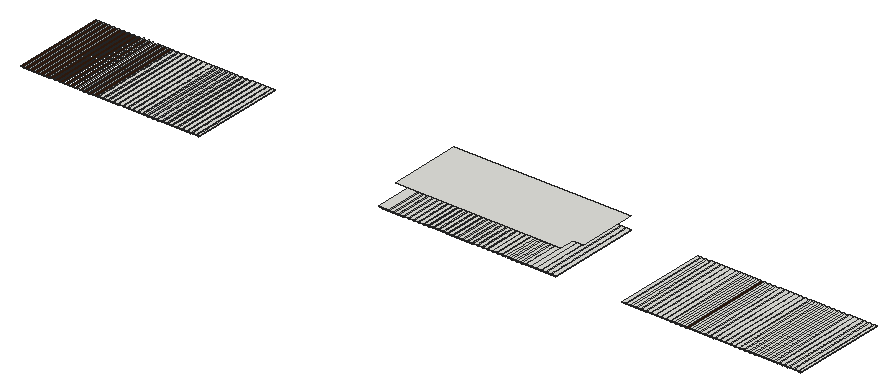
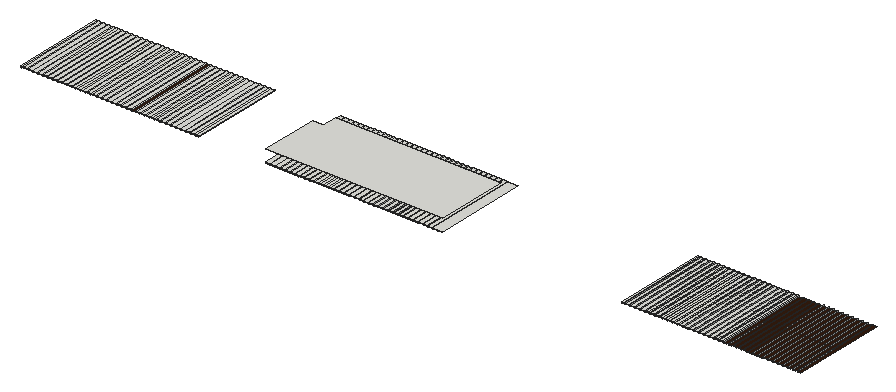
# SketchUp Ruby script. Lengths in inches.
U = 1.inch
M = Sketchup.active_model
def pt(a) = Geom::Point3d.new(a.map { |v| v * U })
def face(e, loops, mat)
  f = e.add_face(loops[0].map { |a| pt(a) })
  loops[1..].each { |l| e.add_face(l.map { |a| pt(a) }).erase! }
  f.material = f.back_material = mat if mat
  f
end
# faces: each face lists its corners as indices into pts; further lists are holes
def faces(e, pts, list, mat = nil) = list.each { |f| face(e, (f[0].is_a?(Array) ? f : [f]).map { |l| l.map { |i| pts[i] } }, mat) }
# xy, xz, yz: faces in a plane at the given z, y or x. An outline is a flat list of corners, or four numbers for a rectangle; further outlines are holes
def ring(l) = l.size == 4 ? [[l[0], l[1]], [l[2], l[1]], [l[2], l[3]], [l[0], l[3]]] : l.each_slice(2).to_a
def flat(e, list, mat, &to3) = list.each { |f| face(e, (f[0].is_a?(Array) ? f : [f]).map { |l| ring(l).map { |u, v| to3.(u, v) } }, mat) }
def xy(e, z, list, mat = nil) = flat(e, list, mat) { |x, y| [x, y, z] }
def xz(e, y, list, mat = nil) = flat(e, list, mat) { |x, z| [x, y, z] }
def yz(e, x, list, mat = nil) = flat(e, list, mat) { |y, z| [x, y, z] }
def lines(e, pts, list) = list.each { |a, b| e.add_line(pt(pts[a]), pt(pts[b])) }
# prism: a flat outline (further loops are holes) pulled along v
def prism(e, loops, v, mat = nil)
  f = face(e, loops, mat); d = Geom::Vector3d.new(v.map { |x| x * U })
  f.pushpull(f.normal.samedirection?(d) ? d.length : -d.length)
end
def box(e, o, s, mat = nil) = prism(e, [[o, [o[0] + s[0], o[1], o[2]], [o[0] + s[0], o[1] + s[1], o[2]], [o[0], o[1] + s[1], o[2]]]], [0, 0, s[2]], mat)
def at(x, y, z, deg = 0) = Geom::Transformation.translation(pt([x, y, z])) * Geom::Transformation.rotation(ORIGIN, Z_AXIS, deg.degrees)
def axes(o, x, y, z) = Geom::Transformation.new([*x, 0, *y, 0, *z, 0, *pt(o).to_a, 1])
def part(name) = M.definitions.add(name)
# library, detail: a bought-in or finely detailed component or shape, given as its bounding box
def library(name, o, s) = part(name).tap { |d| box(d.entities, o, s) }
def detail(e, o, s) = box(e.add_group.entities, o, s)
def put(e, d, t, mat = nil) = e.add_instance(d, t).tap { |i| i.material = mat if mat }
def group(e, t, mat = nil) = e.add_group.tap { |g| g.transformation = t; g.material = mat if mat }.entities
root = M.entities
M.materials.add("[Wood Veneer 01]").color = [51, 28, 15]
xy(root,253.5625,[[1723.81,246.64,1728.56,361.27],[1729.81,246.64,1734.56,361.27],[1735.81,246.64,1740.56,361.27],[1741.81,246.64,1746.56,361.27],[1747.81,246.64,1752.56,361.27],
  [1753.81,246.64,1758.56,361.27],[1759.81,246.64,1764.56,361.27],[1765.81,246.64,1770.56,361.27],[1771.81,246.64,1776.56,361.27],[1777.81,246.64,1782.56,361.27]],"[Wood Veneer 01]")
xy(root,253.875,[[1711.81,246.64,1716.56,361.27],[1717.81,246.64,1722.56,361.27]],"[Wood Veneer 01]")
xy(root,253.9375,[[1130.14,246.64,1134.52,361.27],[1136.14,246.64,1140.52,361.27],[1142.14,246.64,1146.52,361.27],[1148.14,246.64,1152.52,361.27],[1154.14,246.64,1158.52,361.27],
  [1160.14,246.64,1164.52,361.27],[1166.14,246.64,1170.52,361.27],[1172.14,246.64,1176.52,361.27],[1178.14,246.64,1182.52,361.27],[1184.14,246.64,1188.52,361.27],
  [1190.14,246.64,1194.52,361.27],[1196.14,246.64,1200.52,361.27],[1202.14,246.64,1206.52,361.27],[1208.14,246.64,1212.52,361.27],[1214.14,246.64,1218.52,361.27],
  [1220.14,246.64,1224.52,361.27],[1226.14,246.64,1230.52,361.27],[1232.14,246.64,1236.52,361.27],[1238.14,246.64,1242.52,361.27],[1244.14,246.64,1248.52,361.27],
  [1250.14,246.64,1254.52,361.27],[1256.14,246.64,1260.52,361.27],[1262.14,246.64,1266.52,361.27],[1268.14,246.64,1272.52,361.27],[1274.14,246.64,1278.52,361.27],
  [1280.14,246.64,1284.52,361.27],[1286.14,246.64,1290.52,361.27],[1292.14,246.64,1296.52,361.27],[1298.14,246.64,1302.52,361.27],[1304.14,246.64,1308.52,361.27],
  [1310.14,246.64,1314.52,361.27],[1316.14,246.64,1320.52,361.27],[1322.14,246.64,1326.52,361.27],[1328.14,246.64,1332.52,361.27],[1334.14,246.64,1338.52,361.27],
  [1340.14,246.64,1344.52,361.27],[1346.14,246.64,1348.32,361.27],[1567.81,246.64,1572.56,361.27],[1573.81,246.64,1578.56,361.27],[1579.81,246.64,1584.56,361.27],
  [1585.81,246.64,1590.56,361.27],[1591.81,246.64,1596.56,361.27],[1597.81,246.64,1602.56,361.27],[1603.81,246.64,1608.56,361.27],[1609.81,246.64,1614.56,361.27],
  [1615.81,246.64,1620.56,361.27],[1621.81,246.64,1626.56,361.27],[1627.81,246.64,1632.56,361.27],[1633.81,246.64,1638.56,361.27],[1639.81,246.64,1644.56,361.27],
  [1645.81,246.64,1650.56,361.27],[1651.81,246.64,1656.56,361.27],[1657.81,246.64,1662.56,361.27],[1663.81,246.64,1668.56,361.27],[1669.81,246.64,1674.56,361.27],
  [1675.81,246.64,1680.56,361.27],[1681.81,246.64,1686.56,361.27],[1687.81,246.64,1692.56,361.27],[1693.81,246.64,1698.56,361.27],[1699.81,246.64,1704.56,361.27],
  [1705.81,246.64,1710.56,361.27],[1863.7,246.64,1868.08,361.27],[1869.7,246.64,1874.08,361.27],[1875.7,246.64,1880.08,361.27],[1881.7,246.64,1886.08,361.27],
  [1887.7,246.64,1892.08,361.27],[1893.7,246.64,1898.08,361.27],[1899.7,246.64,1904.08,361.27],[1905.7,246.64,1910.08,361.27],[1911.7,246.64,1916.08,361.27],
  [1917.7,246.64,1922.08,361.27],[1923.7,246.64,1928.08,361.27],[1929.7,246.64,1934.08,361.27],[1935.7,246.64,1940.08,361.27],[1941.7,246.64,1946.08,361.27],
  [1947.7,246.64,1952.08,361.27],[1953.7,246.64,1958.08,361.27],[1959.7,246.64,1964.08,361.27],[1965.7,246.64,1970.08,361.27],[1971.7,246.64,1976.08,361.27],
  [1977.7,246.64,1982.08,361.27],[1983.7,246.64,1988.08,361.27],[1989.7,246.64,1994.08,361.27],[1995.7,246.64,2000.08,361.27],[2001.7,246.64,2006.08,361.27],
  [2007.7,246.64,2012.08,361.27],[2013.7,246.64,2018.08,361.27],[2019.7,246.64,2024.08,361.27],[2025.7,246.64,2030.08,361.27],[2031.7,246.64,2036.08,361.27],
  [2037.7,246.64,2042.08,361.27],[2043.7,246.64,2048.08,361.27],[2049.7,246.64,2054.08,361.27],[2055.7,246.64,2060.08,361.27],[2061.7,246.64,2066.08,361.27],
  [2067.7,246.64,2072.08,361.27],[2073.7,246.64,2078.08,361.27],[2079.7,246.64,2081.89,361.27]],"[Wood Veneer 01]")
xy(root,254.625,[[1711.81,246.64,1716.56,361.27]])
xy(root,254.6875,[[1224.52,246.64,1226.14,361.27],[1226.14,246.64,1230.52,361.27],[1230.52,246.64,1232.14,361.27],[1232.14,246.64,1236.52,361.27],[1236.52,246.64,1238.14,361.27],
  [1238.14,246.64,1242.52,361.27],[1242.52,246.64,1244.14,361.27],[1244.14,246.64,1248.52,361.27],[1248.52,246.64,1250.14,361.27],[1250.14,246.64,1254.52,361.27],
  [1254.52,246.64,1256.14,361.27],[1256.14,246.64,1260.52,361.27],[1260.52,246.64,1262.14,361.27],[1262.14,246.64,1266.52,361.27],[1266.52,246.64,1268.14,361.27],
  [1268.14,246.64,1272.52,361.27],[1272.52,246.64,1274.14,361.27],[1274.14,246.64,1278.52,361.27],[1278.52,246.64,1280.14,361.27],[1280.14,246.64,1284.52,361.27],
  [1284.52,246.64,1286.14,361.27],[1286.14,246.64,1290.52,361.27],[1290.52,246.64,1292.14,361.27],[1292.14,246.64,1296.52,361.27],[1296.52,246.64,1298.14,361.27],
  [1298.14,246.64,1302.52,361.27],[1302.52,246.64,1304.14,361.27],[1304.14,246.64,1308.52,361.27],[1308.52,246.64,1310.14,361.27],[1310.14,246.64,1314.52,361.27],
  [1314.52,246.64,1316.14,361.27],[1316.14,246.64,1320.52,361.27],[1320.52,246.64,1322.14,361.27],[1322.14,246.64,1326.52,361.27],[1326.52,246.64,1328.14,361.27],
  [1328.14,246.64,1332.52,361.27],[1332.52,246.64,1334.14,361.27],[1334.14,246.64,1338.52,361.27],[1338.52,246.64,1340.14,361.27],[1340.14,246.64,1344.52,361.27],
  [1344.52,246.64,1346.14,361.27],[1346.14,246.64,1348.32,361.27],[1567.3,246.64,1579.81,361.27],[1579.81,246.64,1584.56,361.27],[1584.56,246.64,1585.81,361.27],
  [1585.81,246.64,1590.56,361.27],[1590.56,246.64,1591.81,361.27],[1591.81,246.64,1596.56,361.27],[1596.56,246.64,1597.81,361.27],[1597.81,246.64,1602.56,361.27],
  [1602.56,246.64,1603.81,361.27],[1603.81,246.64,1608.56,361.27],[1608.56,246.64,1609.81,361.27],[1609.81,246.64,1614.56,361.27],[1614.56,246.64,1615.81,361.27],
  [1615.81,246.64,1620.56,361.27],[1620.56,246.64,1621.81,361.27],[1621.81,246.64,1626.56,361.27],[1626.56,246.64,1627.81,361.27],[1627.81,246.64,1632.56,361.27],
  [1632.56,246.64,1633.81,361.27],[1633.81,246.64,1638.56,361.27],[1638.56,246.64,1639.81,361.27],[1639.81,246.64,1644.56,361.27],[1644.56,246.64,1645.81,361.27],
  [1645.81,246.64,1650.56,361.27],[1650.56,246.64,1651.81,361.27],[1651.81,246.64,1656.56,361.27],[1656.56,246.64,1657.81,361.27],[1657.81,246.64,1662.56,361.27],
  [1662.56,246.64,1663.81,361.27],[1663.81,246.64,1668.56,361.27],[1668.56,246.64,1669.81,361.27],[1669.81,246.64,1674.56,361.27],[1674.56,246.64,1675.81,361.27],
  [1675.81,246.64,1680.56,361.27],[1680.56,246.64,1681.81,361.27],[1681.81,246.64,1686.56,361.27],[1686.56,246.64,1687.81,361.27],[1687.81,246.64,1692.56,361.27],
  [1692.56,246.64,1693.81,361.27],[1693.81,246.64,1698.56,361.27],[1698.56,246.64,1699.81,361.27],[1699.81,246.64,1704.56,361.27],[1704.56,246.64,1705.81,361.27],
  [1705.81,246.64,1710.56,361.27],[1710.56,246.64,1711.81,361.27],[1711.81,246.64,1716.56,361.27],[1716.56,246.64,1717.81,361.27],[1717.81,246.64,1722.56,361.27],
  [1722.56,246.64,1723.81,361.27],[1723.81,246.64,1728.56,361.27],[1728.56,246.64,1729.81,361.27],[1729.81,246.64,1734.56,361.27],[1734.56,246.64,1735.81,361.27],
  [1735.81,246.64,1740.56,361.27],[1740.56,246.64,1741.81,361.27],[1741.81,246.64,1746.56,361.27],[1746.56,246.64,1747.81,361.27],[1747.81,246.64,1752.56,361.27],
  [1752.56,246.64,1753.81,361.27],[1753.81,246.64,1758.56,361.27],[1758.56,246.64,1759.81,361.27],[1759.81,246.64,1764.56,361.27],[1764.56,246.64,1765.81,361.27],
  [1765.81,246.64,1770.56,361.27],[1770.56,246.64,1771.81,361.27],[1771.81,246.64,1776.56,361.27],[1776.56,246.64,1777.81,361.27],[1777.81,246.64,1782.56,361.27],
  [1863.7,246.64,1868.08,361.27],[1868.08,246.64,1869.7,361.27],[1869.7,246.64,1874.08,361.27],[1874.08,246.64,1875.7,361.27],[1875.7,246.64,1880.08,361.27],
  [1880.08,246.64,1881.7,361.27],[1881.7,246.64,1886.08,361.27],[1886.08,246.64,1887.7,361.27],[1887.7,246.64,1892.08,361.27],[1892.08,246.64,1893.7,361.27],
  [1893.7,246.64,1898.08,361.27],[1898.08,246.64,1899.7,361.27],[1899.7,246.64,1904.08,361.27],[1904.08,246.64,1905.7,361.27],[1905.7,246.64,1910.08,361.27],
  [1910.08,246.64,1911.7,361.27],[1911.7,246.64,1916.08,361.27],[1916.08,246.64,1917.7,361.27],[1917.7,246.64,1922.08,361.27],[1922.08,246.64,1923.7,361.27],
  [1923.7,246.64,1928.08,361.27],[1928.08,246.64,1929.7,361.27],[1929.7,246.64,1934.08,361.27],[1934.08,246.64,1935.7,361.27],[1935.7,246.64,1940.08,361.27],
  [1940.08,246.64,1941.7,361.27],[1946.08,246.64,1947.7,361.27],[1947.7,246.64,1952.08,361.27],[1952.08,246.64,1953.7,361.27],[1953.7,246.64,1958.08,361.27],
  [1958.08,246.64,1959.7,361.27],[1959.7,246.64,1964.08,361.27],[1964.08,246.64,1965.7,361.27],[1965.7,246.64,1970.08,361.27],[1970.08,246.64,1971.7,361.27],
  [1971.7,246.64,1976.08,361.27],[1976.08,246.64,1977.7,361.27],[1977.7,246.64,1982.08,361.27],[1982.08,246.64,1983.7,361.27],[1983.7,246.64,1988.08,361.27],
  [1988.08,246.64,1989.7,361.27],[1989.7,246.64,1994.08,361.27],[1994.08,246.64,1995.7,361.27],[1995.7,246.64,2000.08,361.27],[2000.08,246.64,2001.7,361.27],
  [2001.7,246.64,2006.08,361.27],[2006.08,246.64,2007.7,361.27],[2007.7,246.64,2012.08,361.27],[2012.08,246.64,2013.7,361.27],[2013.7,246.64,2018.08,361.27],
  [2018.08,246.64,2019.7,361.27],[2019.7,246.64,2024.08,361.27],[2024.08,246.64,2025.7,361.27],[2025.7,246.64,2030.08,361.27],[2030.08,246.64,2031.7,361.27],
  [2031.7,246.64,2036.08,361.27],[2036.08,246.64,2037.7,361.27],[2037.7,246.64,2042.08,361.27],[2042.08,246.64,2043.7,361.27],[2043.7,246.64,2048.08,361.27],
  [2048.08,246.64,2049.7,361.27],[2049.7,246.64,2054.08,361.27],[2054.08,246.64,2055.7,361.27],[2055.7,246.64,2060.08,361.27],[2060.08,246.64,2061.7,361.27],
  [2061.7,246.64,2066.08,361.27],[2066.08,246.64,2067.7,361.27],[2067.7,246.64,2072.08,361.27],[2072.08,246.64,2073.7,361.27],[2073.7,246.64,2078.08,361.27],
  [2078.08,246.64,2079.7,361.27],[2079.7,246.64,2081.89,361.27]])
xy(root,269.0625,[[1567.3,271.8,1769.03,271.8,1769.03,290.02,1782.56,290.02,1782.56,361.27,1567.3,361.27]])
yz(root,1134.52,[[246.64,253.9375,361.27,254.6875]])
yz(root,1140.52,[[246.64,253.9375,361.27,254.6875]])
yz(root,1146.52,[[246.64,253.9375,361.27,254.6875]])
yz(root,1152.52,[[246.64,253.9375,361.27,254.6875]])
yz(root,1158.52,[[246.64,253.9375,361.27,254.6875]])
yz(root,1164.52,[[246.64,253.9375,361.27,254.6875]])
yz(root,1170.52,[[246.64,253.9375,361.27,254.6875]])
yz(root,1176.52,[[246.64,253.9375,361.27,254.6875]])
yz(root,1182.52,[[246.64,253.9375,361.27,254.6875]])
yz(root,1188.52,[[246.64,253.9375,361.27,254.6875]])
yz(root,1194.52,[[246.64,253.9375,361.27,254.6875]])
yz(root,1200.52,[[246.64,253.9375,361.27,254.6875]])
yz(root,1206.52,[[246.64,253.9375,361.27,254.6875]])
yz(root,1212.52,[[246.64,253.9375,361.27,254.6875]])
yz(root,1218.52,[[246.64,253.9375,361.27,254.6875]])
yz(root,1224.52,[[246.64,253.9375,361.27,254.6875]])
yz(root,1230.52,[[246.64,253.9375,361.27,254.6875]])
yz(root,1236.52,[[246.64,253.9375,361.27,254.6875]])
yz(root,1242.52,[[246.64,253.9375,361.27,254.6875]])
yz(root,1248.52,[[246.64,253.9375,361.27,254.6875]])
yz(root,1254.52,[[246.64,253.9375,361.27,254.6875]])
yz(root,1260.52,[[246.64,253.9375,361.27,254.6875]])
yz(root,1266.52,[[246.64,253.9375,361.27,254.6875]])
yz(root,1272.52,[[246.64,253.9375,361.27,254.6875]])
yz(root,1278.52,[[246.64,253.9375,361.27,254.6875]])
yz(root,1284.52,[[246.64,253.9375,361.27,254.6875]])
yz(root,1290.52,[[246.64,253.9375,361.27,254.6875]])
yz(root,1296.52,[[246.64,253.9375,361.27,254.6875]])
yz(root,1302.52,[[246.64,253.9375,361.27,254.6875]])
yz(root,1308.52,[[246.64,253.9375,361.27,254.6875]])
yz(root,1314.52,[[246.64,253.9375,361.27,254.6875]])
yz(root,1320.52,[[246.64,253.9375,361.27,254.6875]])
yz(root,1326.52,[[246.64,253.9375,361.27,254.6875]])
yz(root,1332.52,[[246.64,253.9375,361.27,254.6875]])
yz(root,1338.52,[[246.64,253.9375,361.27,254.6875]])
yz(root,1344.52,[[246.64,253.9375,361.27,254.6875]])
yz(root,1579.81,[[246.64,253.9375,361.27,254.6875]])
yz(root,1585.81,[[246.64,253.9375,361.27,254.6875]])
yz(root,1591.81,[[246.64,253.9375,361.27,254.6875]])
yz(root,1597.81,[[246.64,253.9375,361.27,254.6875]])
yz(root,1603.81,[[246.64,253.9375,361.27,254.6875]])
yz(root,1609.81,[[246.64,253.9375,361.27,254.6875]])
yz(root,1615.81,[[246.64,253.9375,361.27,254.6875]])
yz(root,1621.81,[[246.64,253.9375,361.27,254.6875]])
yz(root,1627.81,[[246.64,253.9375,361.27,254.6875]])
yz(root,1633.81,[[246.64,253.9375,361.27,254.6875]])
yz(root,1639.81,[[246.64,253.9375,361.27,254.6875]])
yz(root,1645.81,[[246.64,253.9375,361.27,254.6875]])
yz(root,1651.81,[[246.64,253.9375,361.27,254.6875]])
yz(root,1657.81,[[246.64,253.9375,361.27,254.6875]])
yz(root,1663.81,[[246.64,253.9375,361.27,254.6875]])
yz(root,1669.81,[[246.64,253.9375,361.27,254.6875]])
yz(root,1675.81,[[246.64,253.9375,361.27,254.6875]])
yz(root,1681.81,[[246.64,253.9375,361.27,254.6875]])
yz(root,1687.81,[[246.64,253.9375,361.27,254.6875]])
yz(root,1693.81,[[246.64,253.9375,361.27,254.6875]])
yz(root,1699.81,[[246.64,253.9375,361.27,254.6875]])
